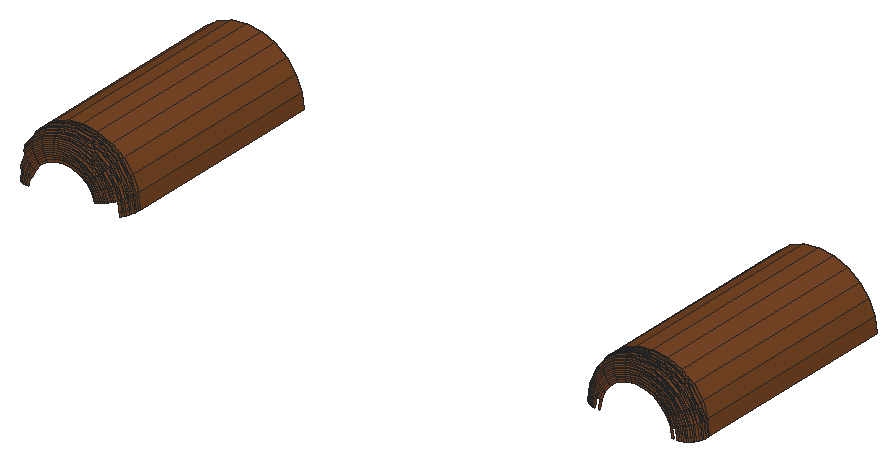
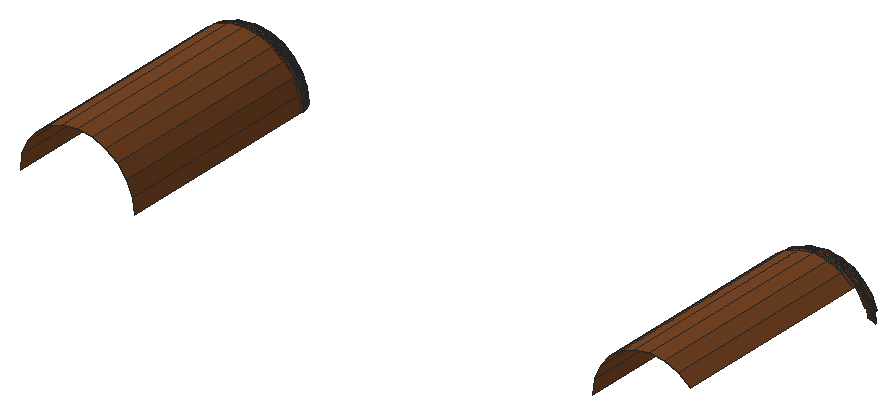
# SketchUp Ruby script. Lengths in inches.
U = 1.inch
M = Sketchup.active_model
def pt(a) = Geom::Point3d.new(a.map { |v| v * U })
def face(e, loops, mat)
  f = e.add_face(loops[0].map { |a| pt(a) })
  loops[1..].each { |l| e.add_face(l.map { |a| pt(a) }).erase! }
  f.material = f.back_material = mat if mat
  f
end
# faces: each face lists its corners as indices into pts; further lists are holes
def faces(e, pts, list, mat = nil) = list.each { |f| face(e, (f[0].is_a?(Array) ? f : [f]).map { |l| l.map { |i| pts[i] } }, mat) }
# xy, xz, yz: faces in a plane at the given z, y or x. An outline is a flat list of corners, or four numbers for a rectangle; further outlines are holes
def ring(l) = l.size == 4 ? [[l[0], l[1]], [l[2], l[1]], [l[2], l[3]], [l[0], l[3]]] : l.each_slice(2).to_a
def flat(e, list, mat, &to3) = list.each { |f| face(e, (f[0].is_a?(Array) ? f : [f]).map { |l| ring(l).map { |u, v| to3.(u, v) } }, mat) }
def xy(e, z, list, mat = nil) = flat(e, list, mat) { |x, y| [x, y, z] }
def xz(e, y, list, mat = nil) = flat(e, list, mat) { |x, z| [x, y, z] }
def yz(e, x, list, mat = nil) = flat(e, list, mat) { |y, z| [x, y, z] }
def lines(e, pts, list) = list.each { |a, b| e.add_line(pt(pts[a]), pt(pts[b])) }
# prism: a flat outline (further loops are holes) pulled along v
def prism(e, loops, v, mat = nil)
  f = face(e, loops, mat); d = Geom::Vector3d.new(v.map { |x| x * U })
  f.pushpull(f.normal.samedirection?(d) ? d.length : -d.length)
end
def box(e, o, s, mat = nil) = prism(e, [[o, [o[0] + s[0], o[1], o[2]], [o[0] + s[0], o[1] + s[1], o[2]], [o[0], o[1] + s[1], o[2]]]], [0, 0, s[2]], mat)
def at(x, y, z, deg = 0) = Geom::Transformation.translation(pt([x, y, z])) * Geom::Transformation.rotation(ORIGIN, Z_AXIS, deg.degrees)
def axes(o, x, y, z) = Geom::Transformation.new([*x, 0, *y, 0, *z, 0, *pt(o).to_a, 1])
def part(name) = M.definitions.add(name)
# library, detail: a bought-in or finely detailed component or shape, given as its bounding box
def library(name, o, s) = part(name).tap { |d| box(d.entities, o, s) }
def detail(e, o, s) = box(e.add_group.entities, o, s)
def put(e, d, t, mat = nil) = e.add_instance(d, t).tap { |i| i.material = mat if mat }
def group(e, t, mat = nil) = e.add_group.tap { |g| g.transformation = t; g.material = mat if mat }.entities
root = M.entities
M.materials.add("[Wood Veneer 01]").color = [120, 70, 37]
xz(root,0,[[60.351,33.683,60.366,33.683,60.377,33.764,60.362,33.768],[60.993,33.683,61.008,33.683,60.997,33.768,60.982,33.764],[55.406,33.756,55.435,33.825,55.419,33.833,55.389,33.761],[55.952,33.756,55.969,33.761,55.939,33.833,55.924,33.825],[60.377,33.764,60.408,33.84,60.395,33.848,60.362,33.768],
  [60.982,33.764,60.997,33.768,60.964,33.848,60.951,33.84],[55.435,33.825,55.48,33.883,55.467,33.896,55.419,33.833],[55.924,33.825,55.939,33.833,55.892,33.896,55.879,33.883],[60.408,33.84,60.458,33.905,60.447,33.916,60.395,33.848],[60.951,33.84,60.964,33.848,60.912,33.916,60.901,33.905],
  [55.48,33.883,55.538,33.928,55.529,33.943,55.467,33.896],[55.879,33.883,55.892,33.896,55.829,33.943,55.821,33.928],[60.458,33.905,60.523,33.955,60.515,33.968,60.447,33.916],[60.901,33.905,60.912,33.916,60.844,33.968,60.836,33.955],[55.538,33.928,55.606,33.956,55.602,33.973,55.529,33.943],
  [55.821,33.928,55.829,33.943,55.757,33.973,55.752,33.956],[60.523,33.955,60.598,33.986,60.594,34.001,60.515,33.968],[60.836,33.955,60.844,33.968,60.764,34.001,60.76,33.986],[55.606,33.956,55.679,33.966,55.679,33.984,55.602,33.973],[55.752,33.956,55.757,33.973,55.679,33.984,55.679,33.966],
  [60.598,33.986,60.679,33.997,60.679,34.012,60.594,34.001],[60.76,33.986,60.764,34.001,60.679,34.012,60.679,33.997]],"[Wood Veneer 01]")
p = [[55.302,0.013,33.683],[55.315,0.013,33.781],[55.302,0.018,33.784],[55.288,0.018,33.683],[55.316,0.009,33.683],[55.328,0.009,33.777],
  [55.33,0.006,33.683],[55.342,0.006,33.774],[55.346,0.003,33.683],[55.357,0.003,33.77],[55.362,0.001,33.683],[55.373,0.001,33.765],
  [55.379,0,33.683],[55.389,0,33.761],[60.234,0.054,33.803],[60.219,0.054,33.683],[60.226,0.046,33.683],[60.241,0.046,33.801],
  [60.234,0.039,33.683],[60.249,0.039,33.799],[60.243,0.032,33.683],[60.258,0.032,33.796],[60.252,0.026,33.683],[60.267,0.026,33.794],
  [60.262,0.021,33.683],[60.276,0.021,33.791],[60.273,0.016,33.683],[60.287,0.016,33.788],[60.284,0.012,33.683],[60.298,0.012,33.786],
  [60.296,0.008,33.683],[60.309,0.008,33.782],[60.309,0.005,33.683],[60.322,0.005,33.779],[60.322,0.003,33.683],[60.334,0.003,33.776],
  [61.024,0.003,33.776],[61.036,0.003,33.683],[61.05,0.005,33.683],[61.037,0.005,33.779],[61.0625,0.008,33.683],[61.049,0.008,33.782],
  [61.074,0.012,33.683],[61.061,0.012,33.786],[61.086,0.016,33.683],[61.072,0.016,33.788],[61.096,0.021,33.683],[61.082,0.021,33.791],
  [61.106,0.026,33.683],[61.092,0.026,33.794],[61.116,0.032,33.683],[61.101,0.032,33.796],[61.125,0.039,33.683],[61.109,0.039,33.799],
  [61.133,0.046,33.683],[61.117,0.046,33.801],[61.14,0.054,33.683],[61.124,0.054,33.803],[56.11,0.054,33.799],[56.125,0.054,33.683],
  [56.134,0.063,33.683],[56.118,0.063,33.801],[56.142,0.073,33.683],[56.126,0.073,33.803],[56.149,0.084,33.683],[56.133,0.084,33.805],
  [56.155,0.096,33.683],[56.139,0.096,33.806],[56.161,0.108,33.683],[56.144,0.108,33.808],[56.166,0.121,33.683],[56.149,0.121,33.809],
  [56.17,0.135,33.683],[56.153,0.135,33.81],[56.173,0.15,33.683],[56.156,0.15,33.811],[56.176,0.165,33.683],[56.159,0.165,33.812],
  [60.198,0.155,33.8125],[60.181,0.155,33.683],[60.182,0.142,33.683],[60.199,0.142,33.812],[60.184,0.128,33.683],[60.201,0.128,33.811],
  [60.1875,0.116,33.683],[60.204,0.116,33.811],[60.191,0.104,33.683],[60.208,0.104,33.81],[60.195,0.093,33.683],[60.212,0.093,33.809],
  [60.2,0.082,33.683],[60.216,0.082,33.807],[60.206,0.072,33.683],[60.222,0.072,33.806],[60.212,0.063,33.683],[60.228,0.063,33.804],
  [61.147,0.063,33.683],[61.131,0.063,33.804],[61.153,0.072,33.683],[61.137,0.072,33.806],[61.159,0.082,33.683],[61.142,0.082,33.807],
  [61.163,0.093,33.683],[61.147,0.093,33.809],[61.168,0.104,33.683],[61.151,0.104,33.81],[61.171,0.116,33.683],[61.154,0.116,33.811],
  [61.174,0.128,33.683],[61.157,0.128,33.811],[61.176,0.142,33.683],[61.159,0.142,33.812],[61.178,0.155,33.683],[61.161,0.155,33.8125],
  [56.178,0.181,33.683],[56.161,0.181,33.8125],[56.179,0.198,33.683],[56.162,0.198,33.8125],[56.179,0.216,33.683],[56.162,0.216,33.813],
  [56.179,2,33.683],[56.162,2,33.813],[60.196,2,33.813],[60.179,2,33.683],[60.179,0.185,33.683],[60.196,0.185,33.813],
  [60.18,0.17,33.683],[60.197,0.17,33.8125],[61.179,0.17,33.683],[61.162,0.17,33.8125],[61.179,0.185,33.683],[61.162,0.185,33.813],
  [61.179,2,33.683],[61.162,2,33.813],[55.29,0.024,33.788],[55.33,0.024,33.885],[55.32,0.03,33.891],[55.278,0.03,33.791],
  [55.341,0.018,33.879],[55.352,0.013,33.872],[55.364,0.009,33.865],[55.377,0.006,33.858],[55.391,0.003,33.85],[55.405,0.001,33.842],
  [55.419,0,33.833],[55.455,0.001,33.908],[55.444,0.003,33.919],[55.467,0,33.896],[55.954,0.001,33.842],[55.904,0.001,33.908],
  [55.892,0,33.896],[55.939,0,33.833],[55.968,0.003,33.85],[55.915,0.003,33.919],[55.986,0.001,33.765],[55.969,0,33.761],
  [56.001,0.003,33.77],[56.016,0.006,33.774],[55.982,0.006,33.858],[56.031,0.009,33.777],[55.994,0.009,33.865],[56.044,0.013,33.781],
  [56.006,0.013,33.872],[56.057,0.018,33.784],[56.018,0.018,33.879],[56.069,0.024,33.788],[56.029,0.024,33.885],[56.08,0.03,33.791],
  [56.039,0.03,33.891],[56.091,0.037,33.794],[56.048,0.037,33.896],[56.101,0.045,33.796],[56.057,0.045,33.901],[56.065,0.054,33.906],
  [60.287,0.046,33.91],[60.28,0.054,33.914],[60.294,0.039,33.906],[60.301,0.032,33.902],[60.309,0.026,33.897],[60.318,0.021,33.892],
  [60.327,0.016,33.886],[60.337,0.012,33.881],[60.348,0.008,33.875],[60.359,0.005,33.869],[60.37,0.003,33.862],[60.348,0.001,33.772],
  [60.382,0.001,33.855],[60.362,0,33.768],[60.395,0,33.848],[60.437,0.001,33.926],[60.447,0,33.916],[60.977,0.001,33.855],
  [60.922,0.001,33.926],[60.912,0,33.916],[60.964,0,33.848],[61.011,0.001,33.772],[60.997,0,33.768],[60.989,0.003,33.862],
  [61,0.005,33.869],[61.011,0.008,33.875],[61.021,0.012,33.881],[61.031,0.016,33.886],[61.041,0.021,33.892],[61.049,0.026,33.897],
  [61.057,0.032,33.902],[61.065,0.039,33.906],[61.072,0.046,33.91],[61.078,0.054,33.914],[56.073,0.063,33.91],[56.08,0.073,33.914],
  [56.086,0.084,33.918],[56.091,0.096,33.921],[56.096,0.108,33.924],[56.101,0.121,33.927],[56.104,0.135,33.929],[56.107,0.15,33.93],
  [56.109,0.165,33.932],[60.249,0.142,33.932],[60.247,0.155,33.933],[60.251,0.128,33.931],[60.253,0.116,33.929],[60.256,0.104,33.927],
  [60.26,0.093,33.925],[60.264,0.082,33.923],[60.269,0.072,33.92],[60.274,0.063,33.917],[61.084,0.063,33.917],[61.09,0.072,33.92],
  [61.094,0.082,33.923],[61.099,0.093,33.925],[61.102,0.104,33.927],[61.105,0.116,33.929],[61.108,0.128,33.931],[61.11,0.142,33.932],
  [61.111,0.155,33.933],[56.111,0.181,33.933],[56.112,0.198,33.933],[56.112,0.216,33.933],[56.112,2,33.933],[60.246,2,33.933],
  [60.246,0.185,33.933],[60.247,0.17,33.933],[61.112,0.17,33.933],[61.112,0.185,33.933],[61.112,2,33.933],[55.302,0.045,33.901],
  [55.371,0.045,33.992],[55.364,0.054,33.998],[55.293,0.054,33.906],[55.31,0.037,33.896],[55.378,0.037,33.985],[55.386,0.03,33.977],
  [55.394,0.024,33.969],[55.403,0.018,33.96],[55.412,0.013,33.95],[55.422,0.009,33.94],[55.433,0.006,33.93],[55.49,0.013,34.01],
  [55.497,0.009,33.998],[55.505,0.006,33.986],[55.513,0.003,33.972],[55.521,0.001,33.958],[55.529,0,33.943],[55.602,0,33.973],
  [55.597,0.001,33.99],[55.757,0,33.973],[55.829,0,33.943],[55.838,0.001,33.958],[55.761,0.001,33.99],[55.846,0.003,33.972],
  [55.926,0.006,33.93],[55.854,0.006,33.986],[55.936,0.009,33.94],[55.861,0.009,33.998],[55.946,0.013,33.95],[55.868,0.013,34.01],
  [55.956,0.018,33.96],[55.965,0.024,33.969],[55.973,0.03,33.977],[55.981,0.037,33.985],[55.988,0.045,33.992],[55.994,0.054,33.998],
  [60.353,0.054,34.009],[60.359,0.046,34.004],[60.364,0.039,33.998],[60.371,0.032,33.992],[60.377,0.026,33.985],[60.384,0.021,33.978],
  [60.392,0.016,33.971],[60.4,0.012,33.963],[60.408,0.008,33.954],[60.417,0.005,33.945],[60.427,0.003,33.936],[60.488,0.008,34.015],
  [60.494,0.005,34.004],[60.501,0.003,33.993],[60.508,0.001,33.981],[60.515,0,33.968],[60.844,0,33.968],[60.851,0.001,33.981],
  [60.932,0.003,33.936],[60.858,0.003,33.993],[60.941,0.005,33.945],[60.865,0.005,34.004],[60.95,0.008,33.954],[60.871,0.008,34.015],
  [60.959,0.012,33.963],[60.967,0.016,33.971],[60.974,0.021,33.978],[60.981,0.026,33.985],[60.988,0.032,33.992],[60.994,0.039,33.998],
  [61,0.046,34.004],[61.005,0.054,34.009],[55.267,0.096,33.921],[55.343,0.096,34.02],[55.339,0.108,34.024],[55.262,0.108,33.924],
  [55.273,0.084,33.918],[55.347,0.084,34.015],[55.279,0.073,33.914],[55.352,0.073,34.01],[55.286,0.063,33.91],[55.358,0.063,34.005],
  [56.001,0.063,34.005],[56.006,0.073,34.01],[56.011,0.084,34.015],[56.016,0.096,34.02],[56.02,0.108,34.024],[56.023,0.121,34.027],
  [56.026,0.135,34.03],[56.029,0.15,34.033],[56.03,0.165,34.034],[60.327,0.155,34.036],[60.328,0.142,34.035],[60.329,0.128,34.033],
  [60.331,0.116,34.031],[60.334,0.104,34.029],[60.337,0.093,34.026],[60.34,0.082,34.022],[60.344,0.072,34.018],[60.349,0.063,34.014],
  [61.01,0.063,34.014],[61.014,0.072,34.018],[61.018,0.082,34.022],[61.022,0.093,34.026],[61.025,0.104,34.029],[61.027,0.116,34.031],
  [61.029,0.128,34.033],[61.031,0.142,34.035],[61.032,0.155,34.036],[56.032,0.181,34.036],[56.033,0.198,34.037],[56.033,0.216,34.037],
  [56.033,2,34.037],[60.326,2,34.037],[60.326,0.185,34.037],[60.326,0.17,34.037],[61.033,0.17,34.037],[61.033,0.185,34.037],
  [61.033,2,34.037],[55.457,0.054,34.069],[55.461,0.045,34.061],[55.466,0.037,34.052],[55.472,0.03,34.043],[55.478,0.024,34.033],
  [55.484,0.018,34.022],[55.572,0.03,34.084],[55.569,0.037,34.095],[55.575,0.024,34.073],[55.578,0.018,34.061],[55.582,0.013,34.048],
  [55.585,0.009,34.035],[55.589,0.006,34.02],[55.593,0.003,34.005],[55.679,0.018,34.074],[55.679,0.013,34.061],[55.679,0.009,34.047],
  [55.679,0.006,34.032],[55.679,0.003,34.017],[55.679,0.001,34.001],[55.679,0,33.984],[55.766,0.003,34.005],[55.77,0.006,34.02],
  [55.773,0.009,34.035],[55.777,0.013,34.048],[55.78,0.018,34.061],[55.875,0.018,34.022],[55.881,0.024,34.033],[55.784,0.024,34.073],
  [55.887,0.03,34.043],[55.787,0.03,34.084],[55.892,0.037,34.052],[55.79,0.037,34.095],[55.897,0.045,34.061],[55.902,0.054,34.069],
  [60.449,0.054,34.082],[60.453,0.046,34.076],[60.457,0.039,34.069],[60.461,0.032,34.061],[60.466,0.026,34.053],[60.471,0.021,34.044],
  [60.476,0.016,34.035],[60.482,0.012,34.025],[60.569,0.026,34.096],[60.571,0.021,34.086],[60.574,0.016,34.076],[60.577,0.012,34.065],
  [60.58,0.008,34.053],[60.583,0.005,34.041],[60.587,0.003,34.028],[60.59,0.001,34.015],[60.594,0,34.001],[60.679,0.008,34.066],
  [60.679,0.005,34.054],[60.679,0.003,34.04],[60.679,0.001,34.027],[60.679,0,34.012],[60.764,0,34.001],[60.768,0.001,34.015],
  [60.772,0.003,34.028],[60.775,0.005,34.041],[60.778,0.008,34.053],[60.877,0.012,34.025],[60.782,0.012,34.065],[60.883,0.016,34.035],
  [60.784,0.016,34.076],[60.888,0.021,34.044],[60.787,0.021,34.086],[60.893,0.026,34.053],[60.79,0.026,34.096],[60.898,0.032,34.061],
  [60.902,0.039,34.069],[60.906,0.046,34.076],[60.91,0.054,34.082],[55.431,0.165,34.113],[55.328,0.165,34.034],[55.33,0.15,34.033],
  [55.432,0.15,34.111],[55.332,0.135,34.03],[55.434,0.135,34.108],[55.335,0.121,34.027],[55.436,0.121,34.105],[55.439,0.108,34.1],
  [55.441,0.096,34.095],[55.445,0.084,34.09],[55.448,0.073,34.084],[55.452,0.063,34.077],[55.906,0.063,34.077],[55.91,0.073,34.084],
  [55.914,0.084,34.09],[55.917,0.096,34.095],[55.92,0.108,34.1],[55.923,0.121,34.105],[55.925,0.135,34.108],[55.926,0.15,34.111],
  [55.928,0.165,34.113],[60.43,0.155,34.115],[60.431,0.142,34.114],[60.432,0.128,34.112],[60.433,0.116,34.109],[60.435,0.104,34.106],
  [60.437,0.093,34.103],[60.44,0.082,34.098],[60.442,0.072,34.094],[60.446,0.063,34.088],[60.913,0.063,34.088],[60.916,0.072,34.094],
  [60.919,0.082,34.098],[60.921,0.093,34.103],[60.923,0.104,34.106],[60.925,0.116,34.109],[60.927,0.128,34.112],[60.928,0.142,34.114],
  [60.929,0.155,34.115],[55.429,2,34.116],[55.326,2,34.037],[55.326,0.216,34.037],[55.429,0.216,34.116],[55.326,0.198,34.037],
  [55.43,0.198,34.116],[55.327,0.181,34.036],[55.43,0.181,34.115],[55.929,0.181,34.115],[55.929,0.198,34.116],[55.929,0.216,34.116],
  [55.929,2,34.116],[60.429,2,34.116],[60.429,0.185,34.116],[60.429,0.17,34.116],[60.929,0.17,34.116],[60.929,0.185,34.116],
  [60.929,2,34.116],[55.566,0.045,34.105],[55.564,0.054,34.114],[55.679,0.054,34.129],[55.679,0.045,34.119],[55.679,0.037,34.109],
  [55.679,0.03,34.098],[55.679,0.024,34.087],[55.792,0.045,34.105],[55.795,0.054,34.114],[60.56,0.054,34.128],[60.562,0.046,34.121],
  [60.564,0.039,34.113],[60.566,0.032,34.105],[60.679,0.054,34.144],[60.679,0.046,34.137],[60.679,0.039,34.129],[60.679,0.032,34.12],
  [60.679,0.026,34.11],[60.679,0.021,34.1],[60.679,0.016,34.09],[60.679,0.012,34.078],[60.792,0.032,34.105],[60.795,0.039,34.113],
  [60.797,0.046,34.121],[60.799,0.054,34.128],[55.551,0.15,34.16],[55.551,0.165,34.163],[55.552,0.135,34.157],[55.553,0.121,34.153],
  [55.555,0.108,34.148],[55.556,0.096,34.143],[55.558,0.084,34.137],[55.56,0.073,34.13],[55.562,0.063,34.122],[55.679,0.121,34.17],
  [55.679,0.108,34.165],[55.679,0.096,34.159],[55.679,0.084,34.153],[55.679,0.073,34.146],[55.679,0.063,34.138],[55.797,0.063,34.122],
  [55.799,0.073,34.13],[55.801,0.084,34.137],[55.802,0.096,34.143],[55.804,0.108,34.148],[55.805,0.121,34.153],[55.806,0.135,34.157],
  [55.807,0.15,34.16],[55.808,0.165,34.163],[60.55,0.155,34.165],[60.551,0.142,34.163],[60.551,0.128,34.161],[60.552,0.116,34.158],
  [60.553,0.104,34.155],[60.554,0.093,34.151],[60.555,0.082,34.146],[60.557,0.072,34.141],[60.558,0.063,34.135],[60.679,0.093,34.167],
  [60.679,0.082,34.163],[60.679,0.072,34.157],[60.679,0.063,34.151],[60.8,0.063,34.135],[60.802,0.072,34.141],[60.803,0.082,34.146],
  [60.805,0.093,34.151],[60.806,0.104,34.155],[60.807,0.116,34.158],[60.807,0.128,34.161],[60.808,0.142,34.163],[60.808,0.155,34.165],
  [55.55,2,34.166],[55.55,0.216,34.166],[55.55,0.198,34.166],[55.55,0.181,34.165],[55.808,0.181,34.165],[55.809,0.198,34.166],
  [55.809,0.216,34.166],[55.809,2,34.166],[60.55,2,34.166],[60.55,0.185,34.166],[60.55,0.17,34.166],[60.809,0.17,34.166],
  [60.809,0.185,34.166],[60.809,2,34.166],[55.679,0.165,34.18],[55.679,0.15,34.177],[55.679,0.135,34.174],[60.679,0.155,34.182],
  [60.679,0.142,34.18],[60.679,0.128,34.178],[60.679,0.116,34.175],[60.679,0.104,34.172],[55.679,2,34.183],[55.679,0.216,34.183],
  [55.679,0.198,34.183],[55.679,0.181,34.182],[60.679,2,34.183],[60.679,0.185,34.183],[60.679,0.17,34.183]]
faces(root,p,[[0,1,2,3],[4,5,1,0],[6,7,5,4],[8,9,7,6],[10,11,9,8],[12,13,11,10],[14,15,16,17],[17,16,18,19],
  [19,18,20,21],[21,20,22,23],[23,22,24,25],[25,24,26,27],[27,26,28,29],[29,28,30,31],[31,30,32,33],[33,32,34,35],
  [36,37,38,39],[39,38,40,41],[41,40,42,43],[43,42,44,45],[45,44,46,47],[47,46,48,49],[49,48,50,51],[51,50,52,53],
  [53,52,54,55],[55,54,56,57],[58,59,60,61],[61,60,62,63],[63,62,64,65],[65,64,66,67],[67,66,68,69],[69,68,70,71],
  [71,70,72,73],[73,72,74,75],[75,74,76,77],[78,79,80,81],[81,80,82,83],[83,82,84,85],[85,84,86,87],[87,86,88,89],
  [89,88,90,91],[91,90,92,93],[93,92,94,95],[95,94,15,14],[57,56,96,97],[97,96,98,99],[99,98,100,101],[101,100,102,103],
  [103,102,104,105],[105,104,106,107],[107,106,108,109],[109,108,110,111],[111,110,112,113],[77,76,114,115],[115,114,116,117],[117,116,118,119],
  [120,121,119,118],[122,123,124,125],[125,124,126,127],[127,126,79,78],[113,112,128,129],[129,128,130,131],[132,133,131,130],[134,135,136,137],
  [2,138,135,134],[1,139,138,2],[5,140,139,1],[7,141,140,5],[9,142,141,7],[11,143,142,9],[13,144,143,11],[143,145,146,142],
  [144,147,145,143],[148,149,150,151],[152,153,149,148],[154,148,151,155],[156,152,148,154],[157,158,152,156],[159,160,158,157],[161,162,160,159],
  [163,164,162,161],[165,166,164,163],[167,168,166,165],[169,170,168,167],[171,172,170,169],[58,173,172,171],[17,174,175,14],[19,176,174,17],
  [21,177,176,19],[23,178,177,21],[25,179,178,23],[27,180,179,25],[29,181,180,27],[31,182,181,29],[33,183,182,31],[35,184,183,33],
  [185,186,184,35],[187,188,186,185],[189,186,188,190],[191,192,193,194],[195,191,194,196],[36,197,191,195],[39,198,197,36],[41,199,198,39],
  [43,200,199,41],[45,201,200,43],[47,202,201,45],[49,203,202,47],[51,204,203,49],[53,205,204,51],[55,206,205,53],[57,207,206,55],
  [61,208,173,58],[63,209,208,61],[65,210,209,63],[67,211,210,65],[69,212,211,67],[71,213,212,69],[73,214,213,71],[75,215,214,73],
  [77,216,215,75],[81,217,218,78],[83,219,217,81],[85,220,219,83],[87,221,220,85],[89,222,221,87],[91,223,222,89],[93,224,223,91],
  [95,225,224,93],[14,175,225,95],[97,226,207,57],[99,227,226,97],[101,228,227,99],[103,229,228,101],[105,230,229,103],[107,231,230,105],
  [109,232,231,107],[111,233,232,109],[113,234,233,111],[115,235,216,77],[117,236,235,115],[119,237,236,117],[121,238,237,119],[239,122,125,240],
  [127,241,240,125],[78,218,241,127],[129,242,234,113],[131,243,242,129],[133,244,243,131],[245,246,247,248],[249,250,246,245],[136,251,250,249],
  [135,252,251,136],[138,253,252,135],[139,254,253,138],[140,255,254,139],[141,256,255,140],[142,146,256,141],[257,254,255,258],[258,255,256,259],
  [259,256,146,260],[260,146,145,261],[261,145,147,262],[262,263,264,261],[265,266,267,268],[266,150,149,267],[267,149,153,269],[269,153,270,271],
  [271,270,272,273],[273,272,274,275],[158,270,153,152],[160,272,270,158],[162,274,272,160],[164,276,274,162],[166,277,276,164],[168,278,277,166],
  [170,279,278,168],[172,280,279,170],[173,281,280,172],[282,175,174,283],[283,174,176,284],[284,176,177,285],[285,177,178,286],[286,178,179,287],
  [287,179,180,288],[288,180,181,289],[289,181,182,290],[290,182,183,291],[291,183,184,292],[292,184,186,189],[293,290,291,294],[294,291,292,295],
  [295,292,189,296],[296,189,190,297],[298,193,192,299],[299,192,300,301],[301,300,302,303],[303,302,304,305],[197,300,192,191],[198,302,300,197],
  [199,304,302,198],[200,306,304,199],[201,307,306,200],[202,308,307,201],[203,309,308,202],[204,310,309,203],[205,311,310,204],[206,312,311,205],
  [207,313,312,206],[314,315,316,317],[318,319,315,314],[320,321,319,318],[322,323,321,320],[248,247,323,322],[208,324,281,173],[209,325,324,208],
  [210,326,325,209],[211,327,326,210],[212,328,327,211],[213,329,328,212],[214,330,329,213],[215,331,330,214],[216,332,331,215],[333,218,217,334],
  [334,217,219,335],[335,219,220,336],[336,220,221,337],[337,221,222,338],[338,222,223,339],[339,223,224,340],[340,224,225,341],[341,225,175,282],
  [226,342,313,207],[227,343,342,226],[228,344,343,227],[229,345,344,228],[230,346,345,229],[231,347,346,230],[232,348,347,231],[233,349,348,232],
  [234,350,349,233],[235,351,332,216],[236,352,351,235],[237,353,352,236],[238,354,353,237],[355,239,240,356],[356,240,241,357],[357,241,218,333],
  [242,358,350,234],[243,359,358,242],[244,360,359,243],[361,247,246,362],[362,246,250,363],[363,250,251,364],[364,251,252,365],[365,252,253,366],
  [366,253,254,257],[364,367,368,363],[365,369,367,364],[366,370,369,365],[257,371,370,366],[258,372,371,257],[259,373,372,258],[260,374,373,259],
  [261,264,374,260],[375,370,371,376],[376,371,372,377],[377,372,373,378],[378,373,374,379],[379,374,264,380],[380,264,263,381],[268,380,381,265],
  [382,379,380,268],[383,378,379,382],[384,377,378,383],[385,376,377,384],[386,375,376,385],[268,267,269,382],[382,269,271,383],[383,271,273,384],
  [384,273,275,385],[385,275,387,386],[386,387,388,389],[389,388,390,391],[391,390,392,393],[275,274,276,387],[387,276,277,388],[388,277,278,390],
  [390,278,279,392],[392,279,280,394],[394,280,281,395],[396,282,283,397],[397,283,284,398],[398,284,285,399],[399,285,286,400],[400,286,287,401],
  [401,287,288,402],[402,288,289,403],[403,289,290,293],[404,400,401,405],[405,401,402,406],[406,402,403,407],[407,403,293,408],[408,293,294,409],
  [409,294,295,410],[410,295,296,411],[411,296,297,412],[413,408,409,414],[414,409,410,415],[415,410,411,416],[416,411,412,417],[417,418,419,416],
  [416,419,420,415],[415,420,421,414],[414,421,422,413],[418,298,299,419],[419,299,301,420],[420,301,303,421],[421,303,305,422],[422,305,423,424],
  [424,423,425,426],[426,425,427,428],[428,427,429,430],[305,304,306,423],[423,306,307,425],[425,307,308,427],[427,308,309,429],[429,309,310,431],
  [431,310,311,432],[432,311,312,433],[433,312,313,434],[435,436,437,438],[438,437,439,440],[440,439,441,442],[442,441,316,443],[443,316,315,444],
  [444,315,319,445],[445,319,321,446],[446,321,323,447],[447,323,247,361],[395,281,324,448],[448,324,325,449],[449,325,326,450],[450,326,327,451],
  [451,327,328,452],[452,328,329,453],[453,329,330,454],[454,330,331,455],[455,331,332,456],[457,333,334,458],[458,334,335,459],[459,335,336,460],
  [460,336,337,461],[461,337,338,462],[462,338,339,463],[463,339,340,464],[464,340,341,465],[465,341,282,396],[434,313,342,466],[466,342,343,467],
  [467,343,344,468],[468,344,345,469],[469,345,346,470],[470,346,347,471],[471,347,348,472],[472,348,349,473],[473,349,350,474],[475,476,477,478],
  [478,477,479,480],[480,479,481,482],[482,481,436,435],[456,332,351,483],[483,351,352,484],[484,352,353,485],[354,486,485,353],[487,355,356,488],
  [488,356,357,489],[489,357,333,457],[474,350,358,490],[490,358,359,491],[360,492,491,359],[362,493,494,361],[363,368,493,362],[495,494,493,496],
  [496,493,368,497],[497,368,367,498],[498,367,369,499],[499,369,370,375],[389,499,375,386],[391,498,499,389],[393,497,498,391],[500,496,497,393],
  [501,495,496,500],[393,392,394,500],[500,394,395,501],[502,396,397,503],[503,397,398,504],[504,398,399,505],[505,399,400,404],[506,502,503,507],
  [507,503,504,508],[508,504,505,509],[509,505,404,510],[510,404,405,511],[511,405,406,512],[512,406,407,513],[513,407,408,413],[413,422,424,513],
  [513,424,426,512],[512,426,428,511],[511,428,430,510],[510,430,514,509],[509,514,515,508],[508,515,516,507],[507,516,517,506],[430,429,431,514],
  [514,431,432,515],[515,432,433,516],[516,433,434,517],[438,518,519,435],[440,520,518,438],[442,521,520,440],[443,522,521,442],[444,523,522,443],
  [445,524,523,444],[446,525,524,445],[447,526,525,446],[361,494,526,447],[527,521,522,528],[528,522,523,529],[529,523,524,530],[530,524,525,531],
  [531,525,526,532],[532,526,494,495],[533,532,495,501],[534,531,532,533],[535,530,531,534],[536,529,530,535],[537,528,529,536],[538,527,528,537],
  [501,395,448,533],[533,448,449,534],[534,449,450,535],[535,450,451,536],[536,451,452,537],[537,452,453,538],[538,453,454,539],[539,454,455,540],
  [540,455,456,541],[542,457,458,543],[543,458,459,544],[544,459,460,545],[545,460,461,546],[546,461,462,547],[547,462,463,548],[548,463,464,549],
  [549,464,465,550],[550,465,396,502],[551,547,548,552],[552,548,549,553],[553,549,550,554],[554,550,502,506],[506,517,555,554],[554,555,556,553],
  [553,556,557,552],[552,557,558,551],[517,434,466,555],[555,466,467,556],[556,467,468,557],[557,468,469,558],[558,469,470,559],[559,470,471,560],
  [560,471,472,561],[561,472,473,562],[562,473,474,563],[564,475,478,565],[480,566,565,478],[482,567,566,480],[435,519,567,482],[541,456,483,568],
  [568,483,484,569],[569,484,485,570],[486,571,570,485],[572,487,488,573],[573,488,489,574],[574,489,457,542],[563,474,490,575],[575,490,491,576],
  [492,577,576,491],[578,519,518,579],[579,518,520,580],[580,520,521,527],[539,580,527,538],[540,579,580,539],[541,578,579,540],[581,542,543,582],
  [582,543,544,583],[583,544,545,584],[584,545,546,585],[585,546,547,551],[551,558,559,585],[585,559,560,584],[584,560,561,583],[583,561,562,582],
  [582,562,563,581],[586,564,565,587],[587,565,566,588],[588,566,567,589],[589,567,519,578],[568,589,578,541],[569,588,589,568],[570,587,588,569],
  [571,586,587,570],[590,572,573,591],[591,573,574,592],[592,574,542,581],[581,563,575,592],[592,575,576,591],[577,590,591,576]],"[Wood Veneer 01]")
